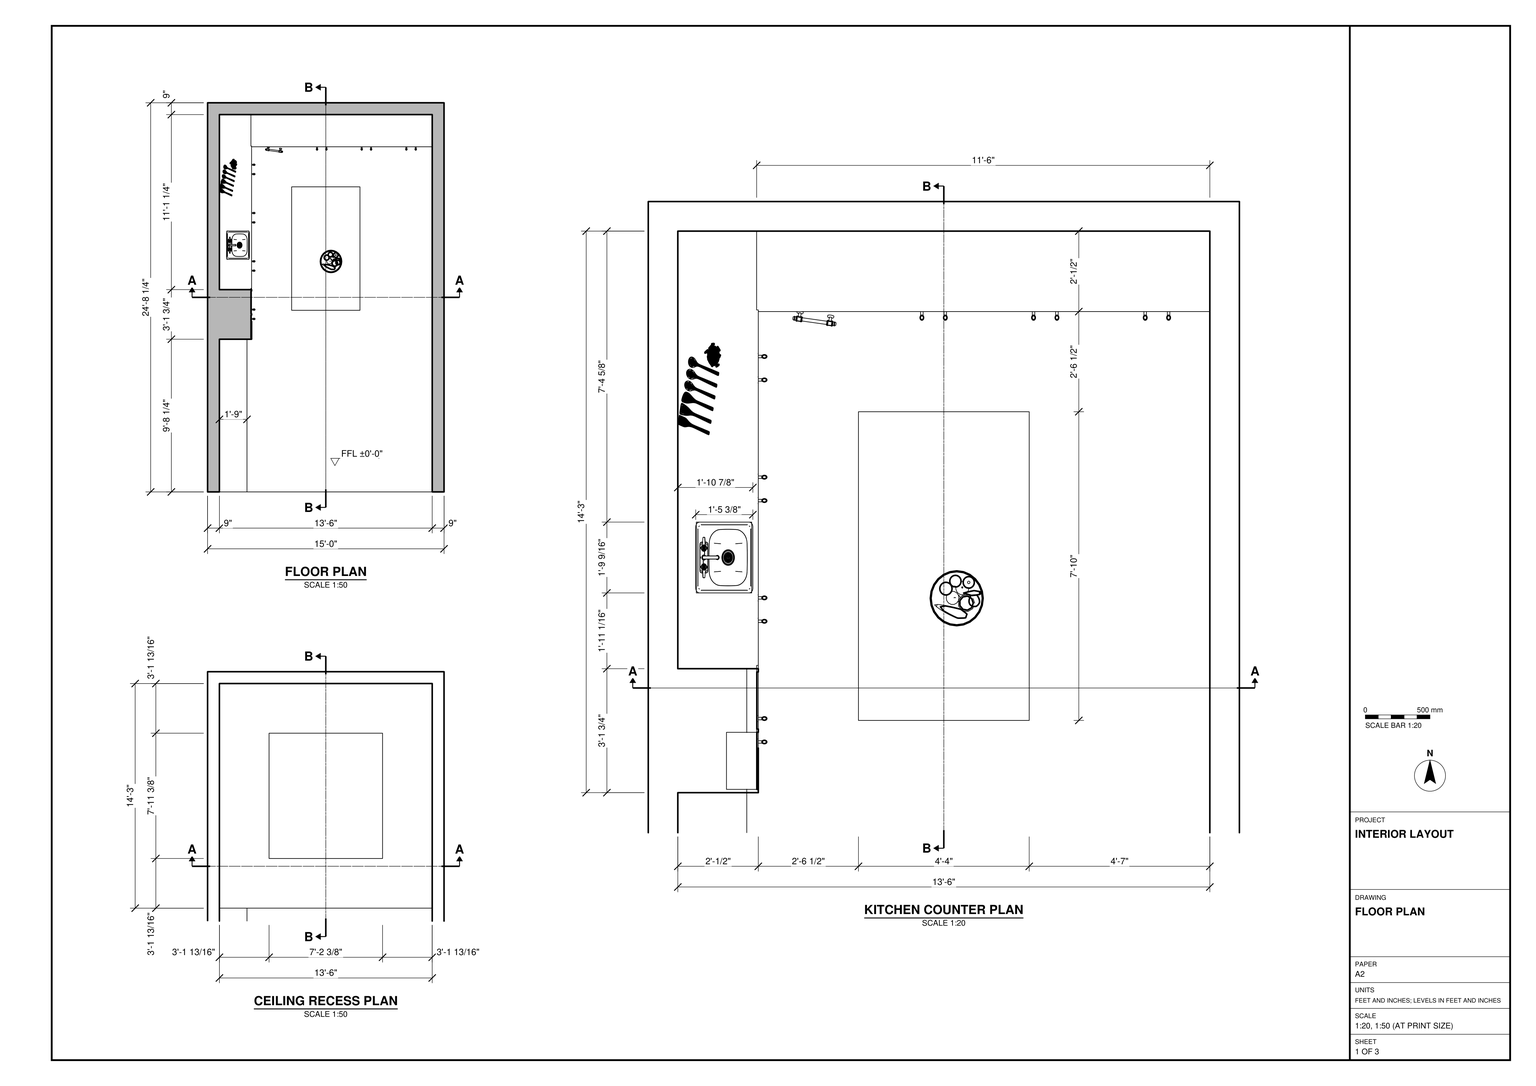
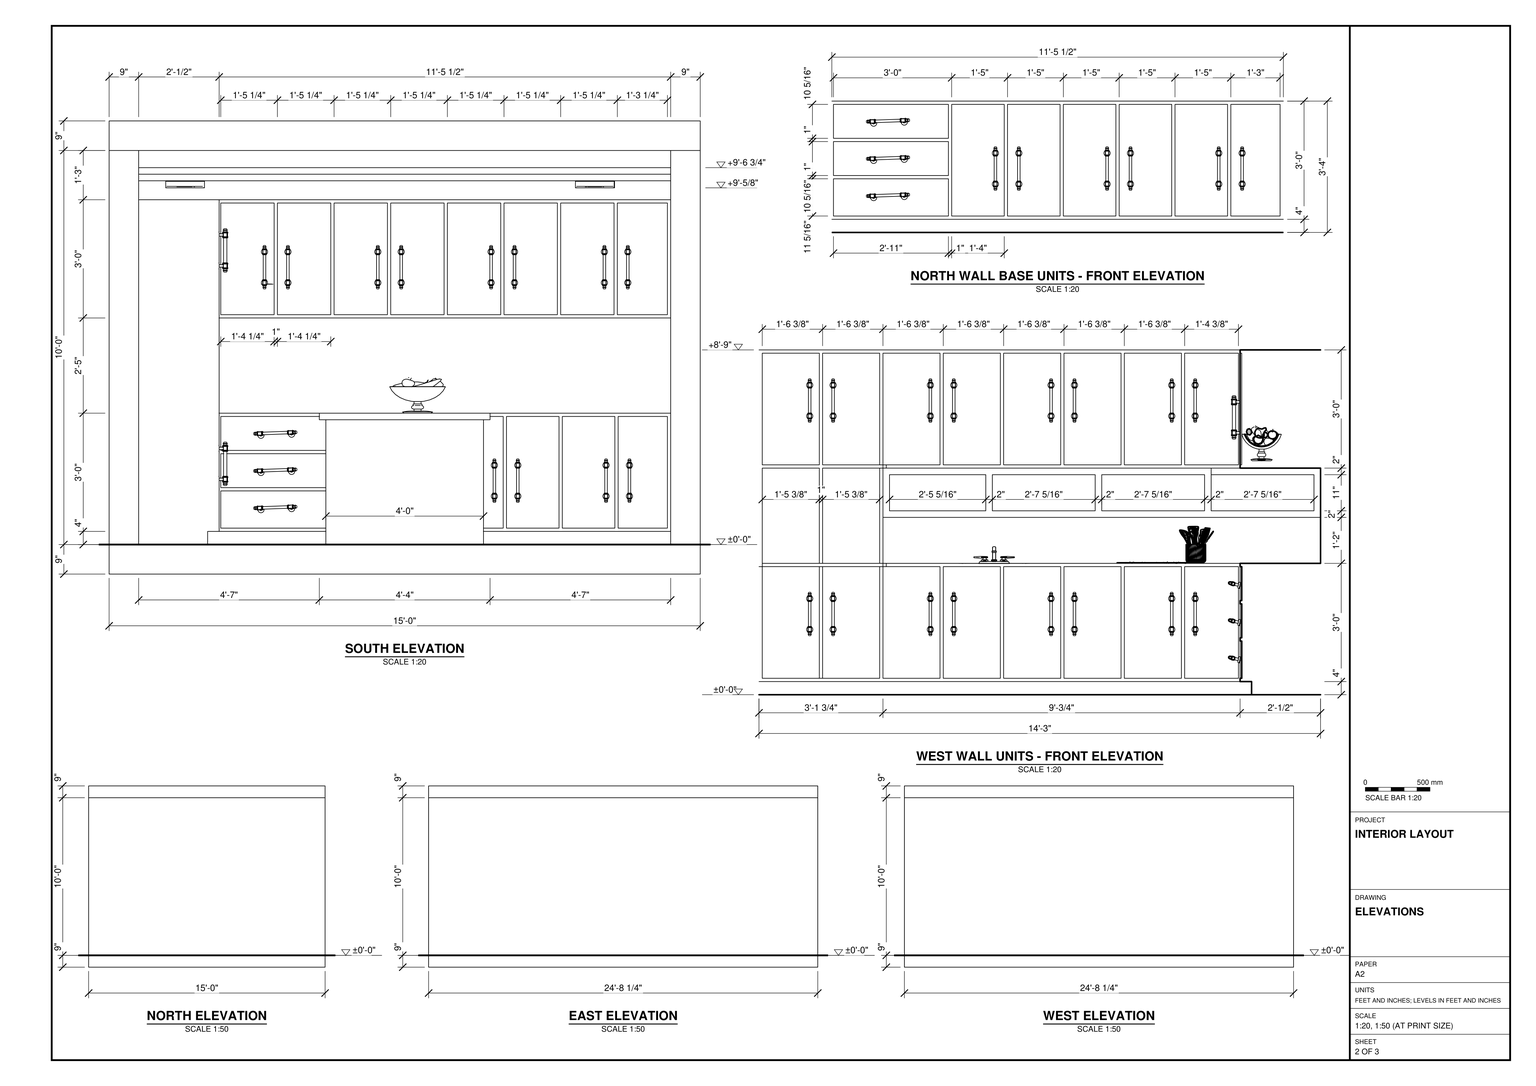
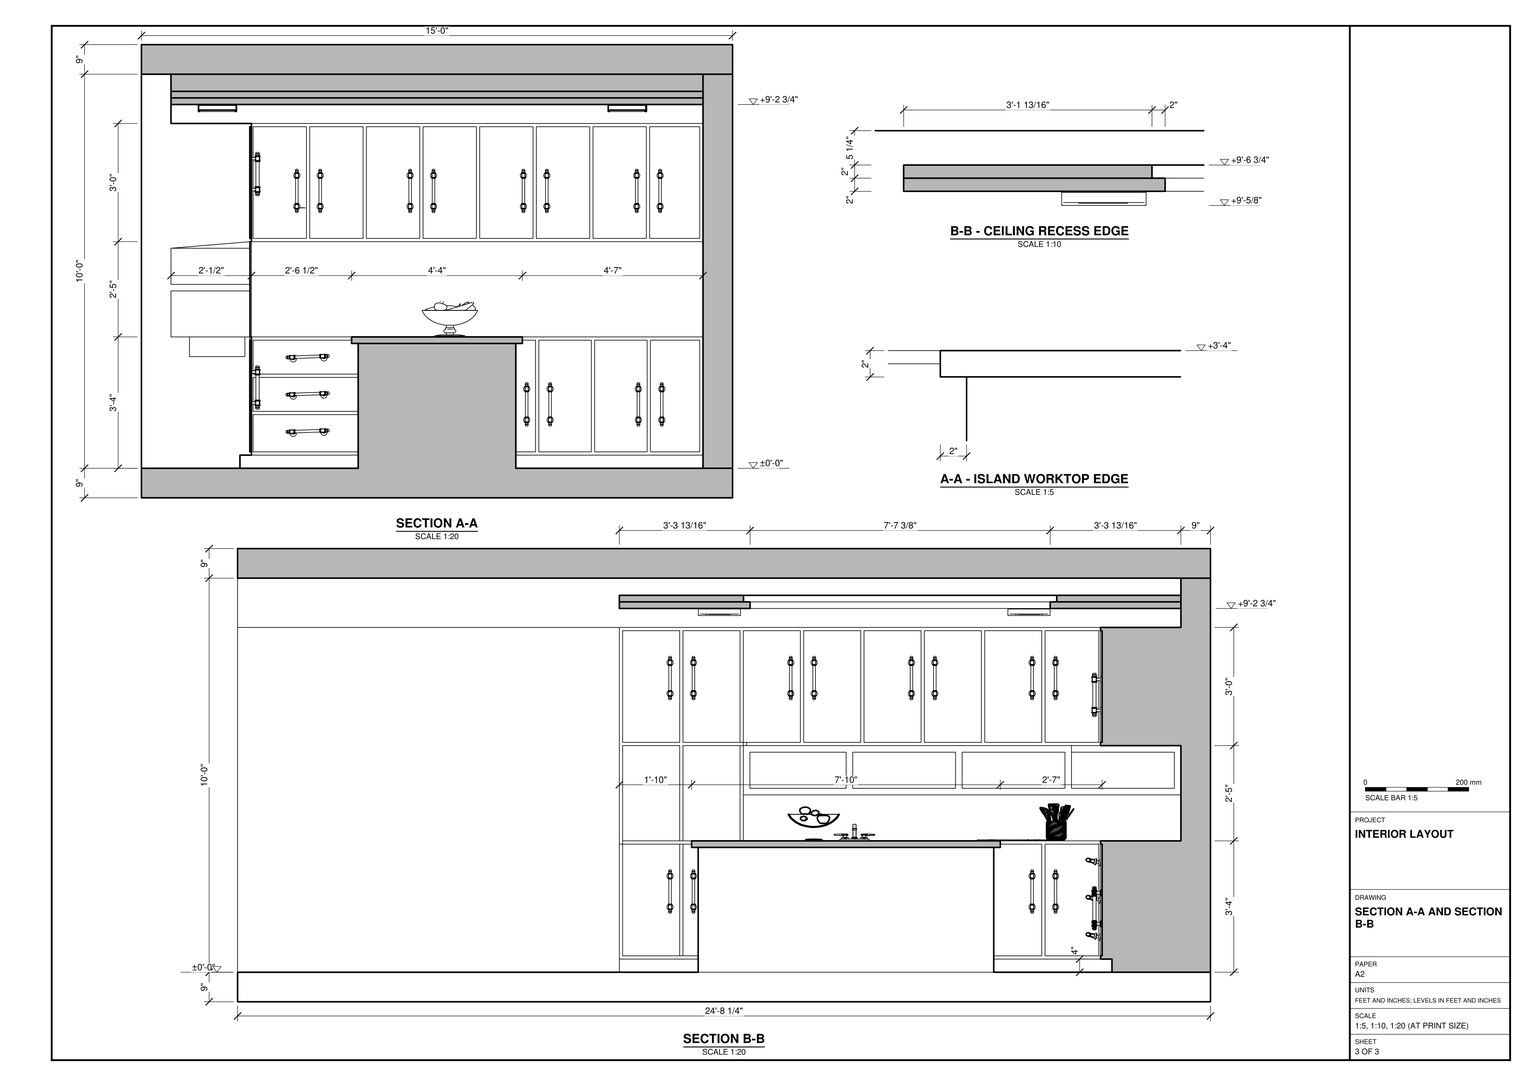
Build the kitchen interior in SketchUp from task_files/diagram_01.pdf, working in feet and inches. The shell is 15'-0" wide, 24'-8 1/4" long and 11'-6" high, with a single finished floor level at ±0'-0". Model the 9" walls on the north, east and west sides and leave the south end open as drawn. Include the floor and roof slabs, each 9" thick.

Use the enlarged counter plan to lay out the kitchen at the north end, leaving the floor area to the south clear. Fit the base and upper cabinets along the north and west walls. Follow the elevations for the plinths, drawer stacks, cupboard doors, pulls and horizontal units above the west counter. Set the sink and faucet into the west run. Place the rectangular island with its long axis running north–south, and use section A-A to form the worktop overhang. Above the island, model the rectangular ceiling recess with the stepped edge shown in section B-B.

Include the bowl on the island, utensils at the west counter and lights at the ceiling recess. Decor and loose items may be any suitable library components, for example from 3D Warehouse. Keep the shell elements and each furniture or joinery piece in separate groups or components, and use components for repeated parts. Save one SketchUp model as output_files/kitchen_with_perimeter_cabinets_and_a_central_island.skp.

# SketchUp Ruby script. Lengths in inches.
U = 1.inch
M = Sketchup.active_model
def pt(a) = Geom::Point3d.new(a.map { |v| v * U })
def face(e, loops, mat)
  f = e.add_face(loops[0].map { |a| pt(a) })
  loops[1..].each { |l| e.add_face(l.map { |a| pt(a) }).erase! }
  f.material = f.back_material = mat if mat
  f
end
# faces: each face lists its corners as indices into pts; further lists are holes
def faces(e, pts, list, mat = nil) = list.each { |f| face(e, (f[0].is_a?(Array) ? f : [f]).map { |l| l.map { |i| pts[i] } }, mat) }
# xy, xz, yz: faces in a plane at the given z, y or x. An outline is a flat list of corners, or four numbers for a rectangle; further outlines are holes
def ring(l) = l.size == 4 ? [[l[0], l[1]], [l[2], l[1]], [l[2], l[3]], [l[0], l[3]]] : l.each_slice(2).to_a
def flat(e, list, mat, &to3) = list.each { |f| face(e, (f[0].is_a?(Array) ? f : [f]).map { |l| ring(l).map { |u, v| to3.(u, v) } }, mat) }
def xy(e, z, list, mat = nil) = flat(e, list, mat) { |x, y| [x, y, z] }
def xz(e, y, list, mat = nil) = flat(e, list, mat) { |x, z| [x, y, z] }
def yz(e, x, list, mat = nil) = flat(e, list, mat) { |y, z| [x, y, z] }
def lines(e, pts, list) = list.each { |a, b| e.add_line(pt(pts[a]), pt(pts[b])) }
# prism: a flat outline (further loops are holes) pulled along v
def prism(e, loops, v, mat = nil)
  f = face(e, loops, mat); d = Geom::Vector3d.new(v.map { |x| x * U })
  f.pushpull(f.normal.samedirection?(d) ? d.length : -d.length)
end
def box(e, o, s, mat = nil) = prism(e, [[o, [o[0] + s[0], o[1], o[2]], [o[0] + s[0], o[1] + s[1], o[2]], [o[0], o[1] + s[1], o[2]]]], [0, 0, s[2]], mat)
def at(x, y, z, deg = 0) = Geom::Transformation.translation(pt([x, y, z])) * Geom::Transformation.rotation(ORIGIN, Z_AXIS, deg.degrees)
def axes(o, x, y, z) = Geom::Transformation.new([*x, 0, *y, 0, *z, 0, *pt(o).to_a, 1])
def part(name) = M.definitions.add(name)
# library, detail: a bought-in or finely detailed component or shape, given as its bounding box
def library(name, o, s) = part(name).tap { |d| box(d.entities, o, s) }
def detail(e, o, s) = box(e.add_group.entities, o, s)
def put(e, d, t, mat = nil) = e.add_instance(d, t).tap { |i| i.material = mat if mat }
def group(e, t, mat = nil) = e.add_group.tap { |g| g.transformation = t; g.material = mat if mat }.entities
root = M.entities
M.materials.add("Emissive").color = [250, 249, 196]
M.materials.add("[0136_Charcoal]").color = [35, 35, 35]
M.materials.add("[Blinds Weave]").color = [141, 91, 25]
M.materials.add("[Marble Carrara Gold Floor Tile]").color = [225, 223, 217]
c1 = library("iron door handle",[0,0,0],[3.91,4.99,27.56])
c2 = library("SINK",[23.25,3.09,31.55],[14.875,14.88,14.9])
c3 = library("CUBIERTOS+DE+MADERA",[-147.91,21.67,0],[150.1,194.68,107.53])
c4 = library("Bowl of Fruit\#1",[0,0,0],[12.07,12.07,13.89])
c5 = part("Group41\#1")
p = [[0,0,0],[0,0,-3.23],[-0.74,0,-3.23],[4.79,-5.65,0],[-4.79,-5.65,0],[4.79,5.65,0],
  [4.79,0,0],[-4.79,5.65,0],[0.74,0,-3.23],[-4.79,0,0],[0,0,-5.22]]
lines(c5.entities,p,[[0,1],[1,2],[3,4],[5,6],[7,5],[1,8],[9,0],[0,6],[8,10],[4,9],[6,3],[2,10],
  [9,7]])
c6 = part("Rectangle Light")
put(c6.entities,c5,at(0,0,0))
c7 = library("Omni Light",[-12,-12,-12],[24,24,24])
c8 = library("Tlon Light 650 Ceiling 152 007",[-12.8,-12.8,-3.78],[25.6,25.6,3.58])
xy(root,-9,[[0,0,180,296.25]])
xy(root,0,[[0,0,9,0,9,116.25,30,116.25,30,266.25,171,266.25,171,0,180,0,180,296.25,0,296.25],[9,0,30,116.25],[[30,0,171,266.25],[66,140.25,114,230.25]]])
xy(root,4,[[30,116.25,33.5,263.25],[33.5,262.75,33.5,263.25,30,263.25,30,266.25,171,266.25,171,262.75]])
xy(root,5,[[23.8125,117.25,33,134.625],[33,117.25,33.5,134.625],[33,135.625,33.5,153],[33,154,33.5,171.375],[33,172.375,33.5,189.75],
  [33,190.75,33.5,208.125],[34,262.75,69,263.25],[70,262.75,86,263.25],[87,262.75,103,263.25],[104,262.75,120,263.25],
  [121,262.75,137,263.25],[138,262.75,154,263.25],[155,262.75,170,263.25]])
xy(root,5,[[33,209.125,33.5,226.5],[33,227.5,33.5,244.875],[33,245.875,33.5,262.25]],"[0136_Charcoal]")
xy(root,16.33,[[34,262.75,69,263.25]])
xy(root,17.33,[[34,262.75,69,263.25]])
xy(root,27.67,[[34,262.75,69,263.25]])
xy(root,28.67,[[34,262.75,69,263.25]])
xy(root,34,[[14.625,177.07,31.5,198.64]],"[Marble Carrara Gold Floor Tile]")
xy(root,38,[[64,138.25,116,140.25],[64,140.25,66,232.25],[66,140.25,114,230.25],[114,140.25,116,232.25],[66,230.25,114,232.25]])
xy(root,39,[[23.8125,117.25,33,134.625],[33,117.25,33.5,134.625],[33,134.625,33.5,135.625],[33,135.625,33.5,153],[33,153,33.5,154],
  [33,154,33.5,155],[33,155,33.5,171.375],[33,172.375,33.5,189.75],[33,190.75,33.5,208.125],[33,209.125,33.5,226.5],
  [33,227.5,33.5,244.875],[33,245.875,33.5,262.25],[34,262.75,69,263.25],[70,262.75,86,263.25],[87,262.75,103,263.25],
  [104,262.75,120,263.25],[121,262.75,137,263.25],[138,262.75,154,263.25],[155,262.75,170,263.25]])
xy(root,40,[[33.0625,117.25,33.5,134.625],[33.0625,135.625,33.5,153],[33,154,33.5,155]])
xy(root,40,[[64,138.25,116,232.25],[[9,154,33,154,33,155,33.5,155,33.5,263.25,33,263.25,33,287.25,9,287.25],[14.625,177.07,31.5,198.64]],[33.5,262.75,171,262.75,171,287.25,33,287.25,33,263.25,33.5,263.25]],"[Marble Carrara Gold Floor Tile]")
xy(root,54,[[9,154,33,285.25],[9,285.25,33,287.25]],"[Marble Carrara Gold Floor Tile]")
xy(root,56,[[9,156,33,185.3125],[9,187.3125,33,218.625],[9,220.625,33,251.9375],[9,253.9375,33,285.25]],"[Marble Carrara Gold Floor Tile]")
xy(root,67,[[9,156,33,185.3125],[9,187.3125,33,218.625],[9,220.625,33,251.9375],[9,253.9375,33,285.25]],"[Marble Carrara Gold Floor Tile]")
xy(root,69,[[33.0625,117.25,33.5,134.125],[33.0625,134.125,33.5,134.625],[33.0625,135.625,33.5,153],[33,154,33.5,263.25],[33.5,262.75,33.5,263.25,33,263.25,33,287.25,171,287.25,171,262.75]])
xy(root,70,[[33,117.25,33.5,134.625],[33,135.625,33.5,153],[33,154,33.5,171.375],[33,172.375,33.5,189.75],[33,190.75,33.5,208.125],
  [33,209.125,33.5,226.5],[33,227.5,33.5,244.875],[33,245.875,33.5,262.25],[34,262.75,50.25,263.25],[51.25,262.75,67.5,263.25],
  [68.5,262.75,84.75,263.25],[85.75,262.75,102,263.25],[103,262.75,119.25,263.25],[120.25,262.75,136.5,263.25],[137.5,262.75,153.75,263.25],
  [154.75,262.75,170,263.25]])
xy(root,104,[[33,117.25,33.5,134.625],[33,135.625,33.5,153],[33,154,33.5,171.375],[34,262.75,50.25,263.25],[51.25,262.75,67.5,263.25],
  [68.5,262.75,84.75,263.25],[85.75,262.75,102,263.25],[103,262.75,119.25,263.25],[120.25,262.75,136.5,263.25],[137.5,262.75,153.75,263.25],
  [154.75,262.75,170,263.25]])
xy(root,104,[[33,172.375,33.5,189.75],[33,190.75,33.5,208.125],[33,209.125,33.5,226.5],[33,227.5,33.5,244.875],[33,245.875,33.5,262.25]],"[0136_Charcoal]")
xy(root,105,[[9,116.25,33.5,116.25,33.5,263.25,33,263.25,33,287.25,9,287.25],[33.5,262.75,171,262.75,171,287.25,33,287.25,33,263.25,33.5,263.25]],"[Marble Carrara Gold Floor Tile]")
xy(root,120,[[0,0,0,296.25,180,296.25,180,0,171,0,171,287.25,9,287.25,9,0],[9,0,171,287.25]])
xy(root,129,[[0,0,180,296.25]])
xz(root,0,[[0,-9,180,0],[0,0,9,120],[171,0,180,120],[0,120,180,129]])
xz(root,116.25,[[9,0,30,0,30,4,33.5,4,33.5,105,9,105]])
xz(root,117.25,[[23.8125,5,33,39],[33,5,33.5,39],[33.0625,40,33.5,41],[33.0625,41,33.5,69],[33,70,33.5,104]])
xz(root,134.625,[[23.8125,5,33,39],[33,5,33.5,39],[33.0625,40,33.5,69],[33,70,33.5,104]])
xz(root,135.625,[[33,5,33.5,39],[33.0625,40,33.5,69],[33,70,33.5,104]])
xz(root,138.25,[[64,38,116,40]])
xz(root,140.25,[[66,0,114,38]],"[Marble Carrara Gold Floor Tile]")
xz(root,153,[[33,5,33.5,39],[33.0625,40,33.5,69],[33,70,33.5,104]])
xz(root,154,[[33,5,33.5,39],[33,39,33.5,40],[9,40,9,54,33,54,33,69,33.5,69,33.5,40],[33,70,33.5,104]])
xz(root,155,[[33,39,33.5,40]])
xz(root,156,[[9,56,33,67]],"[Marble Carrara Gold Floor Tile]")
xz(root,171.375,[[33,5,33.5,39],[33,70,33.5,104]])
xz(root,172.375,[[33,5,33.5,39],[33,70,33.5,104]])
xz(root,177.07,[[14.625,34,31.5,40]],"[Marble Carrara Gold Floor Tile]")
xz(root,185.3125,[[9,56,33,67]],"[Marble Carrara Gold Floor Tile]")
xz(root,187.3125,[[9,56,33,67]],"[Marble Carrara Gold Floor Tile]")
xz(root,189.75,[[33,5,33.5,39],[33,70,33.5,104]],"[0136_Charcoal]")
xz(root,190.75,[[33,5,33.5,39],[33,70,33.5,104]])
xz(root,198.64,[[14.625,34,31.5,40]],"[Marble Carrara Gold Floor Tile]")
xz(root,208.125,[[33,5,33.5,39],[33,70,33.5,104]],"[0136_Charcoal]")
xz(root,209.125,[[33,5,33.5,39],[33,70,33.5,104]])
xz(root,218.625,[[9,56,33,67]],"[Marble Carrara Gold Floor Tile]")
xz(root,220.625,[[9,56,33,67]],"[Marble Carrara Gold Floor Tile]")
xz(root,226.5,[[33,5,33.5,39],[33,70,33.5,104]],"[0136_Charcoal]")
xz(root,227.5,[[33,5,33.5,39],[33,70,33.5,104]])
xz(root,230.25,[[66,0,114,38]])
xz(root,232.25,[[64,38,116,40]])
xz(root,244.875,[[33,5,33.5,39],[33,70,33.5,104]],"[0136_Charcoal]")
xz(root,245.875,[[33,5,33.5,39],[33,70,33.5,104]])
xz(root,251.9375,[[9,56,33,67]],"[Marble Carrara Gold Floor Tile]")
xz(root,253.9375,[[9,56,33,67],[9,67,33,69,33,67]],"[Marble Carrara Gold Floor Tile]")
xz(root,262.25,[[33,5,33.5,39],[33,70,33.5,104]],"[0136_Charcoal]")
xz(root,262.75,[[[33.5,4,171,40],[138,5,154,39],[121,5,137,39],[104,5,120,39],[87,5,103,39],[70,5,86,39],[155,5,170,39],[34,5,69,16.33],[34,28.67,69,39],[34,17.33,69,27.67]],[[33.5,69,171,105],[34,70,50.25,104],[51.25,70,67.5,104],[68.5,70,84.75,104],[85.75,70,102,104],[103,70,119.25,104],[120.25,70,136.5,104],[137.5,70,153.75,104],[154.75,70,170,104]]],"[0136_Charcoal]")
xz(root,263.25,[[34,5,69,16.33],[70,5,86,39],[87,5,103,39],[104,5,120,39],[121,5,137,39],
  [138,5,154,39],[155,5,170,39],[34,17.33,69,27.67],[34,28.67,69,39],[34,70,50.25,104],
  [51.25,70,67.5,104],[68.5,70,84.75,104],[85.75,70,102,104],[103,70,119.25,104],[120.25,70,136.5,104],
  [137.5,70,153.75,104],[154.75,70,170,104]],"[Blinds Weave]")
xz(root,266.25,[[30,0,171,4]])
xz(root,285.25,[[9,56,33,67]],"[Marble Carrara Gold Floor Tile]")
xz(root,287.25,[[9,105,171,120]])
xz(root,287.25,[[9,40,171,40,171,69,33,69,33,54,9,54]],"[Marble Carrara Gold Floor Tile]")
xz(root,296.25,[[0,-9,180,0],[0,0,180,120],[0,120,180,129]])
yz(root,0,[[0,-9,296.25,0],[0,0,296.25,120],[0,120,296.25,129]])
yz(root,9,[[0,0,116.25,105],[0,105,287.25,120]])
yz(root,9,[[154,40,287.25,54],[156,56,185.3125,67],[187.3125,56,218.625,67],[220.625,56,251.9375,67],[253.9375,56,285.25,67]],"[Marble Carrara Gold Floor Tile]")
yz(root,14.625,[[177.07,34,198.64,40]],"[Marble Carrara Gold Floor Tile]")
yz(root,23.8125,[[117.25,5,134.625,39]])
yz(root,30,[[116.25,0,266.25,4]])
yz(root,31.5,[[177.07,34,198.64,40]],"[Marble Carrara Gold Floor Tile]")
yz(root,33,[[117.25,5,134.625,39],[135.625,5,153,39],[154,5,171.375,39],[117.25,70,134.625,104],[135.625,70,153,104],
  [154,70,171.375,104]])
yz(root,33,[[172.375,5,189.75,39],[190.75,5,208.125,39],[209.125,5,226.5,39],[227.5,5,244.875,39],[245.875,5,262.25,39],
  [172.375,70,189.75,104],[190.75,70,208.125,104],[209.125,70,226.5,104],[227.5,70,244.875,104],[245.875,70,262.25,104]],"[Blinds Weave]")
yz(root,33,[[[154,54,287.25,54,287.25,69,253.9375,69,253.9375,67,285.25,67,285.25,56,253.9375,56,253.9375,69,154,69],[220.625,56,251.9375,67],[187.3125,56,218.625,67],[156,56,185.3125,67]]],"[Marble Carrara Gold Floor Tile]")
yz(root,33.0625,[[117.25,40,134.625,69],[135.625,40,153,69]],"[Blinds Weave]")
yz(root,33.5,[[154,39,155,40],[153,40,154,69],[154,69,155,70]])
yz(root,33.5,[[[117.25,5,117.25,69,134.625,69,134.625,40,135.625,40,135.625,69,154,69,154,70,135.625,70,135.625,104,153,104,153,70,154,70,154,104,171.375,104,171.375,70,155,70,155,69,262.75,69,262.75,105,116.25,105,116.25,39,134.625,39,134.625,5],[172.375,70,189.75,104],[190.75,70,208.125,104],[209.125,70,226.5,104],[227.5,70,244.875,104],[117.25,70,134.625,104],[245.875,70,262.25,104]]],"[0136_Charcoal]")
yz(root,33.5,[[[116.25,4,262.75,4,262.75,40,155,40,155,39,171.375,39,171.375,5,154,5,154,40,117.25,40,117.25,39,116.25,39],[172.375,5,189.75,39],[209.125,5,226.5,39],[227.5,5,244.875,39],[190.75,5,208.125,39],[135.625,5,153,39],[245.875,5,262.25,39]],[135.625,5,153,39],[154,5,171.375,39],[117.25,70,134.625,104],[135.625,70,153,104],
  [154,70,171.375,104]],"[Blinds Weave]")
yz(root,34,[[262.75,5,263.25,16.33],[262.75,17.33,263.25,27.67],[262.75,28.67,263.25,39]])
yz(root,34,[[262.75,70,263.25,104]],"[0136_Charcoal]")
yz(root,50.25,[[262.75,70,263.25,104]])
yz(root,51.25,[[262.75,70,263.25,104]],"[0136_Charcoal]")
yz(root,64,[[138.25,38,232.25,40]])
yz(root,66,[[140.25,0,230.25,38]],"[Marble Carrara Gold Floor Tile]")
yz(root,67.5,[[262.75,70,263.25,104]])
yz(root,68.5,[[262.75,70,263.25,104]],"[0136_Charcoal]")
yz(root,69,[[262.75,5,263.25,16.33],[262.75,17.33,263.25,27.67],[262.75,28.67,263.25,39]])
yz(root,70,[[262.75,5,263.25,39]])
yz(root,84.75,[[262.75,70,263.25,104]])
yz(root,85.75,[[262.75,70,263.25,104]],"[0136_Charcoal]")
yz(root,86,[[262.75,5,263.25,39]])
yz(root,87,[[262.75,5,263.25,39]])
yz(root,102,[[262.75,70,263.25,104]])
yz(root,103,[[262.75,5,263.25,39]])
yz(root,103,[[262.75,70,263.25,104]],"[0136_Charcoal]")
yz(root,104,[[262.75,5,263.25,39]])
yz(root,114,[[140.25,0,230.25,38]],"[Marble Carrara Gold Floor Tile]")
yz(root,116,[[138.25,38,232.25,40]])
yz(root,119.25,[[262.75,70,263.25,104]])
yz(root,120,[[262.75,5,263.25,39]])
yz(root,120.25,[[262.75,70,263.25,104]],"[0136_Charcoal]")
yz(root,121,[[262.75,5,263.25,39]])
yz(root,136.5,[[262.75,70,263.25,104]])
yz(root,137,[[262.75,5,263.25,39]])
yz(root,137.5,[[262.75,70,263.25,104]])
yz(root,138,[[262.75,5,263.25,39]])
yz(root,153.75,[[262.75,70,263.25,104]])
yz(root,154,[[262.75,5,263.25,39]])
yz(root,154.75,[[262.75,70,263.25,104]])
yz(root,155,[[262.75,5,263.25,39]])
yz(root,170,[[262.75,5,263.25,39],[262.75,70,263.25,104]])
yz(root,171,[[0,0,0,120,287.25,120,287.25,105,262.75,105,262.75,69,287.25,69,287.25,40,262.75,40,262.75,4,266.25,4,266.25,0]])
yz(root,180,[[0,-9,296.25,0],[0,0,296.25,120],[0,120,296.25,129]])
p = [[33.5,135.625,5],[33.5,134.625,5]]
lines(root,p,[[0,1]])
put(root,c1,axes([46.36,260.06,77.84],[0.4864,0,0],[0,0.64,0],[0,0,0.48]))
put(root,c1,axes([53.49,260.06,77.84],[0.4864,0,0],[0,0.64,0],[0,0,0.48]))
put(root,c1,axes([80.86,260.06,77.84],[0.4864,0,0],[0,0.64,0],[0,0,0.48]))
put(root,c1,axes([87.99,260.06,77.84],[0.4864,0,0],[0,0.64,0],[0,0,0.48]))
put(root,c1,axes([115.36,260.06,77.84],[0.4864,0,0],[0,0.64,0],[0,0,0.48]))
put(root,c1,axes([122.49,260.06,77.84],[0.4864,0,0],[0,0.64,0],[0,0,0.48]))
put(root,c1,axes([149.86,260.06,77.84],[0.4864,0,0],[0,0.64,0],[0,0,0.48]))
put(root,c1,axes([156.99,260.06,77.84],[0.4864,0,0],[0,0.64,0],[0,0,0.48]))
put(root,c1,axes([157.49,260.06,12.84],[0.4864,0,0],[0,0.64,0],[0,0,0.48]))
put(root,c1,axes([150.36,260.06,12.84],[0.4864,0,0],[0,0.64,0],[0,0,0.48]))
put(root,c1,axes([116.36,260.06,12.84],[0.4864,0,0],[0,0.64,0],[0,0,0.48]))
put(root,c1,axes([123.49,260.06,12.84],[0.4864,0,0],[0,0.64,0],[0,0,0.48]))
put(root,c1,axes([82.36,260.06,12.84],[0.4864,0,0],[0,0.64,0],[0,0,0.48]))
put(root,c1,axes([89.49,260.06,12.84],[0.4864,0,0],[0,0.64,0],[0,0,0.48]))
put(root,c1,axes([36.19,130.74,82.96],[0,0.4864,0],[-0.64,0,0],[0,0,0.48]))
put(root,c1,axes([36.19,137.86,82.96],[0,0.4864,0],[-0.64,0,0],[0,0,0.48]))
put(root,c1,axes([36.19,167.49,82.96],[0,0.4864,0],[-0.64,0,0],[0,0,0.48]))
put(root,c1,axes([36.19,174.61,82.96],[0,0.4864,0],[-0.64,0,0],[0,0,0.48]))
put(root,c1,axes([36.19,211.36,82.96],[0,0.4864,0],[-0.64,0,0],[0,0,0.48]))
put(root,c1,axes([36.19,204.24,82.96],[0,0.4864,0],[-0.64,0,0],[0,0,0.48]))
put(root,c1,axes([36.19,240.99,82.96],[0,0.4864,0],[-0.64,0,0],[0,0,0.48]))
put(root,c1,axes([36.19,248.11,82.96],[0,0.4864,0],[-0.64,0,0],[0,0,0.48]))
put(root,c1,axes([36.19,248.11,17.96],[0,0.4864,0],[-0.64,0,0],[0,0,0.48]))
put(root,c1,axes([36.19,240.99,17.96],[0,0.4864,0],[-0.64,0,0],[0,0,0.48]))
put(root,c1,axes([36.19,211.36,17.96],[0,0.4864,0],[-0.64,0,0],[0,0,0.48]))
put(root,c1,axes([36.19,204.24,17.96],[0,0.4864,0],[-0.64,0,0],[0,0,0.48]))
put(root,c1,axes([36.19,174.61,17.96],[0,0.4864,0],[-0.64,0,0],[0,0,0.48]))
put(root,c1,axes([36.19,167.49,17.96],[0,0.4864,0],[-0.64,0,0],[0,0,0.48]))
put(root,c1,axes([36.19,137.86,17.96],[0,0.4864,0],[-0.64,0,0],[0,0,0.48]))
put(root,c1,axes([36.19,130.74,17.96],[0,0.4864,0],[-0.64,0,0],[0,0,0.48]))
put(root,c1,axes([43.93,260.18,34.85],[0.00098,-0.11242,-0.47323],[0.09157,0.61631,-0.14622],[0.47506,-0.0666,0.0168]))
put(root,c1,axes([43.93,260.18,23.52],[0.00098,-0.11242,-0.47323],[0.09157,0.61631,-0.14622],[0.47506,-0.0666,0.0168]))
put(root,c1,axes([43.93,260.18,12.1875],[0.00098,-0.11242,-0.47323],[0.09157,0.61631,-0.14622],[0.47506,-0.0666,0.0168]))
put(root,c2,axes([35.47,143.37,13.73],[0,1.44958,0],[-1.16962,0,0],[0,0,0.67538]))
put(root,c3,axes([9.2,220.875,40],[-0.09356,0,0],[0,0.1564,0],[0,0,0.1054]))
put(root,c4,at(42.09,263.25,71.23))
put(root,c4,axes([85.4375,166.64,40],[1.4065,0,0],[0,1.46,0],[0,0,1]))
put(root,c6,axes([13.27,220.125,54],[-0.89,0,0],[0,11.87617,0],[0,0,1]))
put(root,c7,at(55.875,258.61,56.44))
put(root,c7,at(94.0625,258.61,56.44))
put(root,c7,at(131.3125,258.61,56.44))
put(root,c7,at(55.875,202.86,56.44))
put(root,c7,at(89.75,202.86,56.44))
put(root,c7,at(120.9375,202.86,56.44))
g1 = group(root,at(9,116.25,107.18))
xy(g1,3.59,[[[0,0,162,171],[39.81,39.81,122.19,131.19]]])
xy(g1,5.59,[[[0,0,162,171],[37.81,37.81,124.19,133.19]],[37.81,37.81,39.81,133.19],[39.81,37.81,124.19,39.81],[122.19,39.81,124.19,131.19],[39.81,131.19,124.19,133.19]])
xy(g1,7.59,[[[0,0,162,171],[37.81,37.81,124.19,133.19]],[37.81,37.81,124.19,133.19]])
xz(g1,0,[[0,3.59,162,5.59],[0,5.59,162,7.59]])
xz(g1,39.81,[[39.81,3.59,122.19,5.59]])
xz(g1,131.19,[[39.81,3.59,122.19,5.59]])
xz(g1,171,[[0,3.59,162,5.59],[0,5.59,162,7.59]])
yz(g1,0,[[0,3.59,171,5.59],[0,5.59,171,7.59]])
yz(g1,39.81,[[39.81,3.59,131.19,5.59]])
yz(g1,122.19,[[39.81,3.59,131.19,5.59]])
yz(g1,162,[[0,3.59,171,5.59],[0,5.59,171,7.59]])
put(g1,c8,axes([138.89,30.48,3.7],[0.4608,0,0],[0,0.50232,0],[0,0,0.6]))
put(g1,c8,axes([14.14,30.48,3.7],[0.4608,0,0],[0,0.50232,0],[0,0,0.6]))
put(g1,c8,axes([14.14,124.73,3.7],[0.4608,0,0],[0,0.50232,0],[0,0,0.6]))
put(g1,c8,axes([139.01,124.73,3.7],[0.4608,0,0],[0,0.50232,0],[0,0,0.6]))
g2 = group(g1,at(37.81,37.81,5.59))
xz(g2,0,[[0,0,86.39,2]],"Emissive")
xz(g2,95.39,[[0,0,86.39,2]],"Emissive")
yz(g2,0,[[0,0,95.39,2]],"Emissive")
yz(g2,86.39,[[0,0,95.39,2]],"Emissive")
